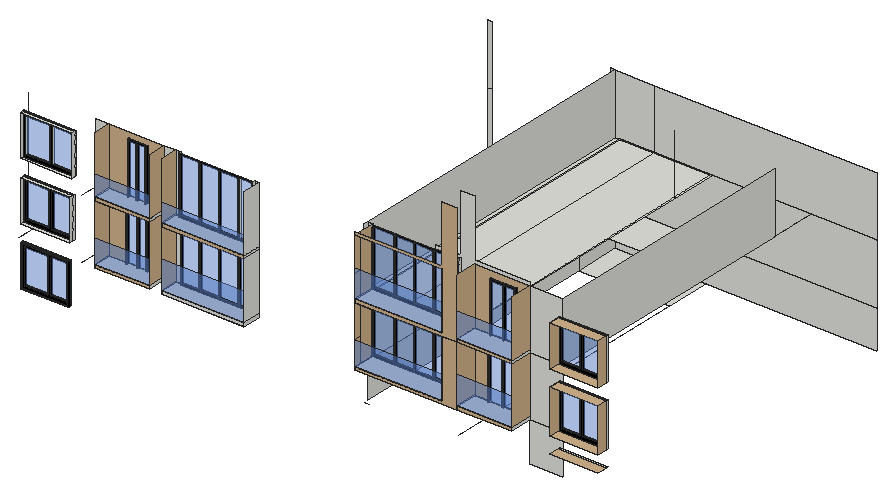
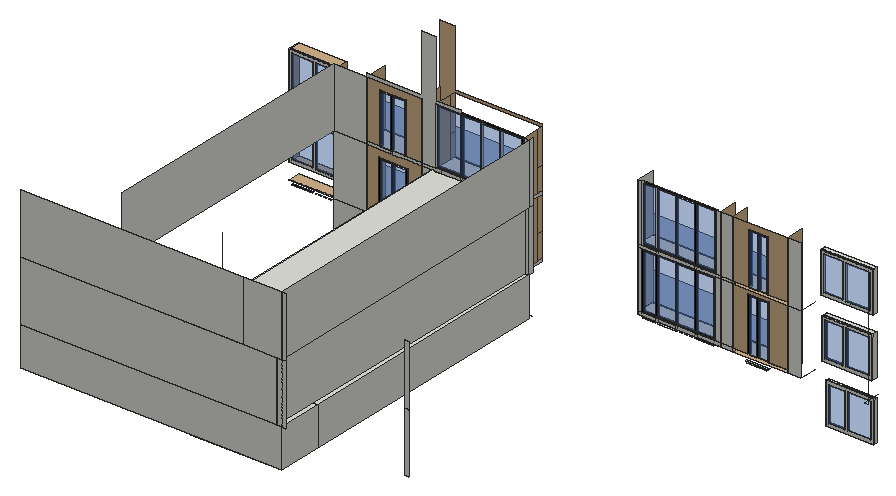
# SketchUp Ruby script. Lengths in inches.
U = 1.inch
M = Sketchup.active_model
def pt(a) = Geom::Point3d.new(a.map { |v| v * U })
def face(e, loops, mat)
  f = e.add_face(loops[0].map { |a| pt(a) })
  loops[1..].each { |l| e.add_face(l.map { |a| pt(a) }).erase! }
  f.material = f.back_material = mat if mat
  f
end
# faces: each face lists its corners as indices into pts; further lists are holes
def faces(e, pts, list, mat = nil) = list.each { |f| face(e, (f[0].is_a?(Array) ? f : [f]).map { |l| l.map { |i| pts[i] } }, mat) }
# xy, xz, yz: faces in a plane at the given z, y or x. An outline is a flat list of corners, or four numbers for a rectangle; further outlines are holes
def ring(l) = l.size == 4 ? [[l[0], l[1]], [l[2], l[1]], [l[2], l[3]], [l[0], l[3]]] : l.each_slice(2).to_a
def flat(e, list, mat, &to3) = list.each { |f| face(e, (f[0].is_a?(Array) ? f : [f]).map { |l| ring(l).map { |u, v| to3.(u, v) } }, mat) }
def xy(e, z, list, mat = nil) = flat(e, list, mat) { |x, y| [x, y, z] }
def xz(e, y, list, mat = nil) = flat(e, list, mat) { |x, z| [x, y, z] }
def yz(e, x, list, mat = nil) = flat(e, list, mat) { |y, z| [x, y, z] }
def lines(e, pts, list) = list.each { |a, b| e.add_line(pt(pts[a]), pt(pts[b])) }
# prism: a flat outline (further loops are holes) pulled along v
def prism(e, loops, v, mat = nil)
  f = face(e, loops, mat); d = Geom::Vector3d.new(v.map { |x| x * U })
  f.pushpull(f.normal.samedirection?(d) ? d.length : -d.length)
end
def box(e, o, s, mat = nil) = prism(e, [[o, [o[0] + s[0], o[1], o[2]], [o[0] + s[0], o[1] + s[1], o[2]], [o[0], o[1] + s[1], o[2]]]], [0, 0, s[2]], mat)
def at(x, y, z, deg = 0) = Geom::Transformation.translation(pt([x, y, z])) * Geom::Transformation.rotation(ORIGIN, Z_AXIS, deg.degrees)
def axes(o, x, y, z) = Geom::Transformation.new([*x, 0, *y, 0, *z, 0, *pt(o).to_a, 1])
def part(name) = M.definitions.add(name)
# library, detail: a bought-in or finely detailed component or shape, given as its bounding box
def library(name, o, s) = part(name).tap { |d| box(d.entities, o, s) }
def detail(e, o, s) = box(e.add_group.entities, o, s)
def put(e, d, t, mat = nil) = e.add_instance(d, t).tap { |i| i.material = mat if mat }
def group(e, t, mat = nil) = e.add_group.tap { |g| g.transformation = t; g.material = mat if mat }.entities
root = M.entities
M.materials.add("[0035_Tan]").color = [210, 180, 140]
M.materials.add("[0137_Black]").color = [0, 0, 0]
M.materials.add("[Translucent Glass Blue]").color = [100, 149, 237]
M.materials["[Translucent Glass Blue]"].alpha = 0.5
xy(root,157.15,[[83.625,162.2,178.82,165.57],[83.625,165.57,178.82,168.57]])
xy(root,163.15,[[89.625,165.57,135,168.57],[140.93,165.57,172.82,168.57]],"[0137_Black]")
xy(root,168.8125,[[737.47,731.95,917.4,821.88]])
xy(root,226.47,[[1141.77,183.2,1177.52,186.2],[1183.52,183.2,1225.27,186.2]],"[0137_Black]")
xy(root,229.5625,[[985.28,204.2,1008.35,207.2],[1011.35,204.2,1031.41,207.2]],"[0137_Black]")
xy(root,232.4,[[89.625,165.57,135,168.57],[140.93,165.57,172.82,168.57]])
xy(root,232.47,[[1135.77,183.2,1231.27,186.2]])
xy(root,232.47,[[1135.77,162.2,1231.27,183.2]],"[0035_Tan]")
xy(root,232.5625,[[982.28,204.2,1034.41,207.2]],"[0137_Black]")
xy(root,235.3125,[[271.43,195.2,290.12,198.2],[292.87,195.2,311.93,198.2]])
xy(root,238.3125,[[268.43,195.2,314.93,198.2]])
xy(root,238.4,[[83.625,162.2,178.82,165.57],[83.625,165.57,178.82,168.57]])
xy(root,243,[[415.22,195.2,451.16,198.2],[454.16,195.2,484.28,198.2],[484.28,195.2,489.53,198.2],[492.53,195.2,517.76,198.2]])
xy(root,243,[[378.57,195.2,412.22,198.2],[751.75,204.2,793,207.2],[796,204.2,831.1875,207.2],[834.1875,204.2,870.375,207.2],[873.375,204.2,911.73,207.2],
  [911.73,204.2,918.86,207.2]],"[0137_Black]")
xy(root,246,[[364.125,162.2,364.125,198.2,375.57,198.2,375.57,195.2,520.76,195.2,520.76,198.2,528.5625,198.2,528.5625,162.2],[921.86,162.2,930.34,199.63],[930.34,162.2,950.28,199.63],[375.57,195.2,412.22,198.2],[412.22,195.2,415.22,198.2],
  [415.22,195.2,451.16,198.2],[451.16,195.2,454.16,198.2],[454.16,195.2,489.53,198.2],[489.53,195.2,492.53,198.2],[492.53,195.2,520.76,198.2],
  [737.47,198.2,748.75,207.2],[921.86,199.63,930.34,207.2],[930.34,199.63,950.28,207.2],[748.75,204.2,793,207.2],[793,204.2,796,207.2],
  [796,204.2,831.1875,207.2],[831.1875,204.2,834.1875,207.2],[834.1875,204.2,870.375,207.2],[870.375,204.2,873.375,207.2],[873.375,204.2,911.73,207.2],
  [911.73,204.2,921.86,207.2],[737.47,207.2,746.47,731.95],[737.47,731.95,746.47,821.88],[746.47,731.95,930.34,821.88]])
xy(root,246,[[231.59,162.2,340.0625,198.2],[748.75,162.2,921.86,204.2],[950.28,162.2,1060.15,207.2]],"[0035_Tan]")
xy(root,252,[[231.59,162.2,340.0625,162.2,340.0625,198.2,309.85,198.2,309.85,195.2,306.85,195.2,306.85,198.2,292.57,198.2,292.57,195.2,288.7,195.2,288.7,198.2,270.54,198.2,270.54,195.2,267.54,195.2,267.54,198.2,231.59,198.2],[364.125,162.2,528.5625,162.2,528.5625,198.2,520.39,198.2,520.39,195.2,375.32,195.2,375.32,198.2,364.125,198.2],[748.75,162.2,921.86,204.2],[950.28,162.2,1060.15,162.2,1060.15,207.2,1035.75,207.2,1035.75,204.2,1032.75,204.2,1032.75,207.2,1010.53,207.2,1010.53,204.2,1007.53,204.2,1007.53,207.2,982.31,207.2,982.31,204.2,979.31,204.2,979.31,207.2,950.28,207.2],[375.32,195.2,412.22,198.2],
  [412.22,195.2,415.22,198.2],[415.22,195.2,451.16,198.2],[451.16,195.2,454.16,198.2],[454.16,195.2,489.53,198.2],[489.53,195.2,492.53,198.2],
  [492.53,195.2,520.39,198.2],[748.75,204.2,793,207.2],[793,204.2,796,207.2],[796,204.2,831.1875,207.2],[831.1875,204.2,834.1875,207.2],
  [834.1875,204.2,870.375,207.2],[870.375,204.2,873.375,207.2],[873.375,204.2,911.73,207.2],[911.73,204.2,921.86,207.2],[979.31,204.2,982.31,207.2],
  [1007.53,204.2,1008.35,207.2],[1008.35,204.2,1010.53,207.2],[1032.75,204.2,1035.75,207.2]])
xy(root,255,[[378.32,195.2,412.22,198.2],[415.22,195.2,451.16,198.2],[454.16,195.2,489.53,198.2],[492.53,195.2,517.39,198.2],[751.75,204.2,793,207.2],
  [796,204.2,831.1875,207.2],[834.1875,204.2,870.375,207.2],[873.375,204.2,911.73,207.2],[911.73,204.2,918.86,207.2]],"[0137_Black]")
xy(root,264.66,[[1135.77,183.2,1231.27,186.2]])
xy(root,264.66,[[1135.77,162.2,1231.27,183.2]],"[0035_Tan]")
xy(root,270.66,[[1141.77,183.2,1177.52,186.2],[1183.52,183.2,1225.27,186.2]],"[0137_Black]")
xy(root,273.03,[[83.625,162.2,182.53,169.82],[83.625,169.82,182.53,172.82]])
xy(root,279.03,[[89.625,169.82,134.93,172.82],[140.93,169.82,176.53,172.82]],"[0137_Black]")
xy(root,345.78,[[1141.77,183.2,1177.52,186.2],[1183.52,183.2,1225.27,186.2]],"[0137_Black]")
xy(root,348.1875,[[982.31,204.2,1007.53,207.2],[1010.53,204.2,1032.75,207.2]])
xy(root,348.28,[[89.625,169.82,134.93,172.82],[140.93,169.82,176.53,172.82]])
xy(root,351.1875,[[979.31,204.2,1035.75,207.2]],"[0137_Black]")
xy(root,351.78,[[1135.77,183.2,1231.27,186.2]])
xy(root,351.78,[[1135.77,162.2,1231.27,183.2]],"[0035_Tan]")
xy(root,354.28,[[83.625,162.2,182.53,169.82],[83.625,169.82,182.53,172.82]])
xy(root,356.5625,[[270.54,195.2,288.7,198.2],[292.57,195.2,306.85,198.2]],"[0137_Black]")
xy(root,359.5625,[[267.54,195.2,309.85,198.2]],"[0137_Black]")
xy(root,363,[[378.32,195.2,412.22,198.2],[415.22,195.2,451.16,198.2],[454.16,195.2,484.28,198.2],[484.28,195.2,489.53,198.2],[492.53,195.2,517.39,198.2],
  [751.75,204.2,793,207.2],[796,204.2,814.9,207.2],[814.9,204.2,831.1875,207.2],[834.1875,204.2,870.375,207.2],[873.375,204.2,911.73,207.2],
  [911.73,204.2,918.86,207.2]],"[0137_Black]")
xy(root,366,[[921.86,162.2,928.15,207.2],[928.15,162.2,930.34,207.2],[930.34,162.2,950.28,207.2],[375.32,195.2,412.22,198.2],[412.22,195.2,415.22,198.2],
  [415.22,195.2,489.53,198.2],[489.53,195.2,492.53,198.2],[492.53,195.2,520.39,198.2],[748.75,204.2,793,207.2],[793,204.2,796,207.2],
  [796,204.2,814.9,207.2],[814.9,204.2,831.1875,207.2],[831.1875,204.2,834.1875,207.2],[834.1875,204.2,870.375,207.2],[870.375,204.2,873.375,207.2],
  [873.375,204.2,911.73,207.2],[911.73,204.2,921.86,207.2],[737.47,207.2,746.47,821.88],[746.47,207.2,814.9,821.88],[814.9,207.2,928.15,821.88],
  [928.15,207.2,930.34,731.95],[928.15,731.95,930.34,821.88]])
xy(root,366,[[231.59,162.2,340.0625,198.2],[364.125,162.2,364.125,198.2,375.32,198.2,375.32,195.2,520.39,195.2,520.39,198.2,528.5625,198.2,528.5625,162.2],[748.75,162.2,921.86,174.2],[950.28,162.2,1060.15,207.2],[748.75,174.2,921.86,204.2]],"[0035_Tan]")
xy(root,372,[[231.59,162.2,340.0625,162.2,340.0625,198.2,308.39,198.2,308.39,195.2,305.39,195.2,305.39,198.2,290.52,198.2,290.52,195.2,287.52,195.2,287.52,198.2,272.83,198.2,272.83,195.2,269.83,195.2,269.83,198.2,231.59,198.2],[364.125,162.2,528.5625,162.2,528.5625,198.2,519.88,198.2,519.88,195.2,372.82,195.2,372.82,198.2,364.125,198.2],[748.75,162.2,921.86,204.2],[950.28,162.2,1060.15,162.2,1060.15,207.2,1034.41,207.2,1034.41,204.2,1031.41,204.2,1031.41,207.2,1011.35,207.2,1011.35,204.2,1008.35,204.2,1008.35,207.2,985.28,207.2,985.28,204.2,982.28,204.2,982.28,207.2,950.28,207.2],[372.82,195.2,412.22,198.2],
  [412.22,195.2,415.22,198.2],[415.22,195.2,489.53,198.2],[489.53,195.2,492.53,198.2],[492.53,195.2,519.88,198.2],[748.75,204.2,793,207.2],
  [793,204.2,796,207.2],[796,204.2,831.1875,207.2],[831.1875,204.2,834.1875,207.2],[834.1875,204.2,870.375,207.2],[870.375,204.2,873.375,207.2],
  [873.375,204.2,911.73,207.2],[911.73,204.2,921.86,207.2],[982.28,204.2,985.28,207.2],[1008.35,204.2,1011.35,207.2],[1031.41,204.2,1034.41,207.2]])
xy(root,375,[[911.73,204.2,918.86,207.2]])
xy(root,375,[[375.82,195.2,412.22,198.2],[415.22,195.2,451.16,198.2],[454.16,195.2,489.53,198.2],[492.53,195.2,516.88,198.2],[751.75,204.2,793,207.2],
  [796,204.2,831.1875,207.2],[834.1875,204.2,870.375,207.2],[873.375,204.2,911.73,207.2]],"[0137_Black]")
xy(root,383.34,[[1135.77,183.2,1231.27,186.2]])
xy(root,383.34,[[1135.77,162.2,1231.27,183.2]],"[0035_Tan]")
xy(root,388.91,[[83.625,162.2,186.23,168.95],[83.625,168.95,186.23,171.95]])
xy(root,389.34,[[1141.77,183.2,1177.52,186.2],[1183.52,183.2,1225.27,186.2]],"[0137_Black]")
xy(root,394.91,[[89.625,168.95,137.0625,171.95],[142.78,168.95,180.23,171.95]])
xy(root,460.47,[[1141.77,183.2,1177.52,186.2],[1183.52,183.2,1225.27,186.2]],"[0137_Black]")
xy(root,464.16,[[89.625,168.95,137.0625,171.95],[142.78,168.95,180.23,171.95]])
xy(root,466.47,[[1135.77,183.2,1231.27,186.2]])
xy(root,466.47,[[1135.77,162.2,1231.27,183.2]],"[0035_Tan]")
xy(root,468.9375,[[985.28,204.2,1008.35,207.2],[1011.35,204.2,1031.41,207.2]])
xy(root,470.16,[[83.625,162.2,186.23,168.95],[83.625,168.95,186.23,171.95]])
xy(root,471.9375,[[982.28,204.2,1034.41,207.2]])
xy(root,471.9375,[[272.83,195.2,287.52,198.2],[290.52,195.2,305.39,198.2]],"[0137_Black]")
xy(root,474.9375,[[269.83,195.2,308.39,198.2]],"[0137_Black]")
xy(root,483,[[375.82,195.2,412.22,198.2],[415.22,195.2,451.16,198.2],[454.16,195.2,484.28,198.2],[484.28,195.2,489.53,198.2],[492.53,195.2,516.88,198.2]])
xy(root,483,[[751.75,204.2,793,207.2],[796,204.2,814.9,207.2],[814.9,204.2,831.1875,207.2],[834.1875,204.2,870.375,207.2],[873.375,204.2,911.73,207.2],
  [911.73,204.2,918.86,207.2]],"[0137_Black]")
xz(root,162.2,[[364.125,246,528.5625,252]])
xz(root,162.2,[[231.59,246,340.0625,252],[748.75,246,950.28,246,950.28,366,921.86,366,921.86,252,748.75,252],[950.28,246,1060.15,252],[231.59,366,340.0625,372],[364.125,366,528.5625,372],
  [748.75,366,950.28,366,950.28,606,921.86,606,921.86,492,748.75,492,748.75,486,921.86,486,921.86,372,748.75,372],[950.28,366,1060.15,372]],"[0035_Tan]")
xz(root,162.2,[[231.59,252,340.0625,299.77],[364.125,252,528.5625,309],[748.75,252,921.86,300.08],[950.28,252,1060.15,309],[231.59,372,340.0625,413.33],
  [364.125,372,528.5625,409.78],[748.75,372,921.86,428],[950.28,372,1060.15,422.45]],"[Translucent Glass Blue]")
xz(root,165.57,[[[83.625,157.15,178.82,238.4],[89.625,163.15,135,232.4],[140.93,163.15,172.82,232.4]]],"[0137_Black]")
xz(root,168.57,[[[83.625,157.15,178.82,238.4],[89.625,163.15,135,232.4],[140.93,163.15,172.82,232.4]]])
xz(root,168.57,[[89.625,163.15,135,232.4],[140.93,163.15,172.82,232.4]],"[Translucent Glass Blue]")
xz(root,168.95,[[[83.625,388.91,186.23,470.16],[89.625,394.91,137.0625,464.16],[142.78,394.91,180.23,464.16]]],"[0137_Black]")
xz(root,169.82,[[[83.625,273.03,182.53,354.28],[89.625,279.03,134.93,348.28],[140.93,279.03,176.53,348.28]]],"[0137_Black]")
xz(root,171.95,[[[83.625,388.91,186.23,470.16],[89.625,394.91,137.0625,464.16],[142.78,394.91,180.23,464.16]]])
xz(root,171.95,[[89.625,394.91,137.0625,464.16],[142.78,394.91,180.23,464.16]],"[Translucent Glass Blue]")
xz(root,172.82,[[[83.625,273.03,182.53,354.28],[89.625,279.03,134.93,348.28],[140.93,279.03,176.53,348.28]]])
xz(root,172.82,[[89.625,279.03,134.93,348.28],[140.93,279.03,176.53,348.28]],"[Translucent Glass Blue]")
xz(root,183.2,[[[1135.77,264.66,1231.27,351.78],[1183.52,270.66,1225.27,345.78],[1141.77,270.66,1177.52,345.78]],[[1135.77,383.34,1231.27,466.47],[1183.52,389.34,1225.27,460.47],[1141.77,389.34,1177.52,460.47]]],"[0137_Black]")
xz(root,186.2,[[[1135.77,264.66,1231.27,351.78],[1183.52,270.66,1225.27,345.78],[1141.77,270.66,1177.52,345.78]],[[1135.77,383.34,1231.27,466.47],[1183.52,389.34,1225.27,460.47],[1141.77,389.34,1177.52,460.47]]])
xz(root,186.2,[[1141.77,270.66,1177.52,345.78],[1183.52,270.66,1225.27,345.78],[1141.77,389.34,1177.52,460.47],[1183.52,389.34,1225.27,460.47]],"[Translucent Glass Blue]")
xz(root,195.2,[[267.54,252,270.54,252,270.54,356.5625,288.7,356.5625,288.7,252,292.57,252,292.57,356.5625,306.85,356.5625,306.85,252,309.85,252,309.85,359.5625,267.54,359.5625],[[375.32,252,520.39,366],[415.22,255,451.16,363],[454.16,255,489.53,363],[378.32,255,412.22,363],[492.53,255,517.39,363]],[269.83,372,272.83,372,272.83,471.9375,287.52,471.9375,287.52,372,290.52,372,290.52,471.9375,305.39,471.9375,305.39,372,308.39,372,308.39,474.9375,269.83,474.9375],[[372.82,372,519.88,486],[375.82,375,412.22,483],[415.22,375,451.16,483],[454.16,375,489.53,483],[492.53,375,516.88,483]]],"[0137_Black]")
xz(root,198.2,[[204.84,246,231.59,366],[340.0625,246,364.125,252],[364.125,246,412.22,252],[412.22,246,415.22,252],[415.22,246,451.16,252],
  [451.16,246,454.16,252],[454.16,246,489.53,252],[489.53,246,492.53,252],[492.53,246,528.5625,252],[340.0625,252,364.125,366],
  [364.125,252,375.32,366],[520.39,252,528.5625,366],[204.84,366,231.59,486],[340.0625,366,364.125,372],[364.125,366,412.22,372],
  [412.22,366,415.22,372],[415.22,366,489.53,372],[489.53,366,492.53,372],[492.53,366,528.5625,372],[340.0625,372,364.125,486],
  [364.125,372,372.82,486],[519.88,372,528.5625,486]])
xz(root,198.2,[[231.59,252,267.54,252,267.54,359.5625,309.85,359.5625,309.85,252,340.0625,252,340.0625,366,231.59,366],[231.59,372,269.83,372,269.83,474.9375,308.39,474.9375,308.39,372,340.0625,372,340.0625,486,231.59,486]],"[0035_Tan]")
xz(root,198.2,[[270.54,252,288.7,356.5625],[292.57,252,306.85,356.5625],[378.32,255,412.22,363],[415.22,255,451.16,363],[454.16,255,489.53,363],
  [492.53,255,517.39,363],[272.83,372,287.52,471.9375],[290.52,372,305.39,471.9375],[375.82,375,412.22,483],[415.22,375,451.16,483],
  [454.16,375,489.53,483],[492.53,375,516.88,483]],"[Translucent Glass Blue]")
xz(root,204.2,[[[748.75,252,921.86,366],[873.375,255,918.86,363],[751.75,255,793,363],[834.1875,255,870.375,363],[796,255,831.1875,363]],[979.31,252,982.31,252,982.31,348.1875,1007.53,348.1875,1007.53,252,1010.53,252,1010.53,348.1875,1032.75,348.1875,1032.75,252,1035.75,252,1035.75,351.1875,979.31,351.1875],[[748.75,372,921.86,486],[873.375,375,918.86,483],[751.75,375,793,483],[834.1875,375,870.375,483],[796,375,831.1875,483]],[982.28,372,985.28,372,985.28,468.9375,1008.35,468.9375,1008.35,372,1011.35,372,1011.35,468.9375,1031.41,468.9375,1031.41,372,1034.41,372,1034.41,471.9375,982.28,471.9375]],"[0137_Black]")
xz(root,207.2,[[1060.15,168.8125,1125.97,246],[737.47,246,746.47,366],[746.47,246,748.75,366],[748.75,246,793,252],[793,246,796,252],
  [796,246,831.1875,252],[831.1875,246,834.1875,252],[834.1875,246,870.375,252],[870.375,246,873.375,252],[873.375,246,911.73,252],
  [911.73,246,911.73,252,921.86,252,921.86,366,950.28,366,950.28,246],[950.28,246,1008.35,252],[1008.35,246,1011.35,252],[1011.35,246,1060.15,252],[1060.15,246,1125.97,366],
  [737.47,366,748.75,486],[748.75,366,793,372],[793,366,796,372],[796,366,831.1875,372],[831.1875,366,834.1875,372],
  [834.1875,366,870.375,372],[870.375,366,873.375,372],[873.375,366,911.73,372],[911.73,366,950.28,372],[950.28,366,1008.35,372],
  [1008.35,366,1011.35,372],[1011.35,366,1060.15,372],[1060.15,366,1125.97,486],[921.86,372,950.28,372,950.28,486,1060.15,486,1060.15,492,950.28,492,950.28,606,921.86,606,921.86,492,873.375,492,873.375,486,921.86,486]])
xz(root,207.2,[[950.28,252,979.31,252,979.31,351.1875,1035.75,351.1875,1035.75,252,1060.15,252,1060.15,366,950.28,366],[950.28,372,982.28,372,982.28,471.9375,1034.41,471.9375,1034.41,372,1060.15,372,1060.15,486,950.28,486]],"[0035_Tan]")
xz(root,207.2,[[982.31,252,1007.53,348.1875],[1010.53,252,1032.75,348.1875],[751.75,255,793,363],[796,255,831.1875,363],[834.1875,255,870.375,363],
  [873.375,255,918.86,363],[985.28,372,1008.35,468.9375],[1011.35,372,1031.41,468.9375],[751.75,375,793,483],[796,375,831.1875,483],
  [834.1875,375,870.375,483],[873.375,375,918.86,483]],"[Translucent Glass Blue]")
xz(root,821.88,[[737.47,168.8125,1256.59,246],[484.28,246,493.28,366],[728.47,246,737.47,366],[737.47,246,746.47,366],[746.47,246,1256.59,366],
  [484.28,366,493.28,486],[728.47,366,737.47,486],[737.47,366,814.9,486],[814.9,366,1256.59,486]])
yz(root,83.625,[[162.2,157.15,165.57,238.4],[165.57,157.15,168.57,238.4],[162.2,273.03,169.82,354.28],[169.82,273.03,172.82,354.28],[162.2,388.91,168.95,470.16],
  [168.95,388.91,171.95,470.16]])
yz(root,89.625,[[168.95,394.91,171.95,464.16]])
yz(root,89.625,[[165.57,163.15,168.57,232.4],[169.82,279.03,172.82,348.28]],"[0137_Black]")
yz(root,134.93,[[169.82,279.03,172.82,348.28]],"[0137_Black]")
yz(root,135,[[165.57,163.15,168.57,232.4]],"[0137_Black]")
yz(root,137.0625,[[168.95,394.91,171.95,464.16]])
yz(root,140.93,[[165.57,163.15,168.57,232.4],[169.82,279.03,172.82,348.28]],"[0137_Black]")
yz(root,142.78,[[168.95,394.91,171.95,464.16]])
yz(root,172.82,[[165.57,163.15,168.57,232.4]],"[0137_Black]")
yz(root,176.53,[[169.82,279.03,172.82,348.28]],"[0137_Black]")
yz(root,178.82,[[165.57,157.15,168.57,238.4]])
yz(root,178.82,[[162.2,157.15,165.57,238.4]],"[0137_Black]")
yz(root,180.23,[[168.95,394.91,171.95,464.16]])
yz(root,182.53,[[162.2,273.03,169.82,354.28],[169.82,273.03,172.82,354.28]])
yz(root,186.23,[[162.2,388.91,168.95,470.16],[168.95,388.91,171.95,470.16]])
yz(root,231.59,[[162.2,246,198.2,252],[162.2,366,198.2,372]])
yz(root,231.59,[[162.2,252,198.2,366],[162.2,372,198.2,486]],"[0035_Tan]")
yz(root,267.54,[[195.2,252,198.2,359.5625]],"[0137_Black]")
yz(root,269.83,[[195.2,372,198.2,474.9375]],"[0137_Black]")
yz(root,270.54,[[195.2,252,198.2,356.5625]],"[0137_Black]")
yz(root,272.83,[[195.2,372,198.2,375]])
yz(root,272.83,[[195.2,375,198.2,471.9375]],"[0137_Black]")
yz(root,287.52,[[195.2,372,198.2,471.9375]],"[0137_Black]")
yz(root,288.7,[[195.2,252,198.2,356.5625]],"[0137_Black]")
yz(root,290.52,[[195.2,372,198.2,471.9375]],"[0137_Black]")
yz(root,292.57,[[195.2,252,198.2,356.5625]],"[0137_Black]")
yz(root,305.39,[[195.2,372,198.2,375]])
yz(root,305.39,[[195.2,375,198.2,471.9375]],"[0137_Black]")
yz(root,306.85,[[195.2,252,198.2,356.5625]],"[0137_Black]")
yz(root,308.39,[[195.2,372,198.2,474.9375]],"[0137_Black]")
yz(root,309.85,[[195.2,252,198.2,359.5625]],"[0137_Black]")
yz(root,340.0625,[[162.2,246,198.2,252],[162.2,366,198.2,372]])
yz(root,340.0625,[[162.2,252,198.2,366],[162.2,372,198.2,486]],"[0035_Tan]")
yz(root,364.125,[[162.2,246,198.2,252],[162.2,366,198.2,372]])
yz(root,364.125,[[162.2,252,198.2,366],[162.2,372,198.2,486]],"[0035_Tan]")
yz(root,372.82,[[195.2,372,198.2,486]])
yz(root,375.32,[[195.2,252,198.2,366]],"[0137_Black]")
yz(root,375.82,[[195.2,375,198.2,483]],"[0137_Black]")
yz(root,378.32,[[195.2,255,198.2,363]],"[0137_Black]")
yz(root,412.22,[[195.2,255,198.2,363],[195.2,375,198.2,483]],"[0137_Black]")
yz(root,415.22,[[195.2,255,198.2,363],[195.2,375,198.2,483]],"[0137_Black]")
yz(root,451.16,[[195.2,255,198.2,363],[195.2,375,198.2,483]],"[0137_Black]")
yz(root,454.16,[[195.2,255,198.2,363],[195.2,375,198.2,483]],"[0137_Black]")
yz(root,489.53,[[195.2,255,198.2,363],[195.2,375,198.2,483]],"[0137_Black]")
yz(root,492.53,[[195.2,375,198.2,483]])
yz(root,492.53,[[195.2,255,198.2,363]],"[0137_Black]")
yz(root,516.88,[[195.2,375,198.2,483]],"[0137_Black]")
yz(root,517.39,[[195.2,255,198.2,363]],"[0137_Black]")
yz(root,519.88,[[195.2,372,198.2,486]])
yz(root,520.39,[[195.2,252,198.2,366]],"[0137_Black]")
yz(root,528.5625,[[162.2,246,198.2,252],[162.2,252,198.2,366],[162.2,366,198.2,372],[162.2,372,198.2,486]])
yz(root,737.47,[[207.2,168.8125,731.95,246],[731.95,168.8125,821.88,246],[198.2,246,207.2,366],[198.2,366,207.2,486],[207.2,366,821.88,486]])
yz(root,746.47,[[207.2,246,821.88,366]])
yz(root,748.75,[[162.2,246,198.2,252],[198.2,246,207.2,252],[204.2,252,207.2,366],[162.2,366,198.2,372],[198.2,366,207.2,372],
  [204.2,372,207.2,486]])
yz(root,748.75,[[162.2,252,174.2,300.08],[174.2,252,204.2,366],[162.2,300.08,174.2,366],[162.2,372,174.2,416.46],[174.2,372,204.2,486],
  [162.2,416.46,174.2,486]],"[0035_Tan]")
yz(root,751.75,[[204.2,255,207.2,363],[204.2,375,207.2,483]],"[0137_Black]")
yz(root,793,[[204.2,375,207.2,483]])
yz(root,793,[[204.2,255,207.2,363]],"[0137_Black]")
yz(root,796,[[204.2,255,207.2,363],[204.2,375,207.2,483]],"[0137_Black]")
yz(root,831.1875,[[204.2,375,207.2,483]])
yz(root,831.1875,[[204.2,255,207.2,363]],"[0137_Black]")
yz(root,834.1875,[[204.2,255,207.2,363],[204.2,375,207.2,483]],"[0137_Black]")
yz(root,870.375,[[204.2,255,207.2,363],[204.2,375,207.2,483]],"[0137_Black]")
yz(root,873.375,[[204.2,255,207.2,363],[204.2,375,207.2,483]],"[0137_Black]")
yz(root,918.86,[[204.2,255,207.2,363],[204.2,375,207.2,483]],"[0137_Black]")
yz(root,921.86,[[204.2,252,207.2,366],[204.2,372,207.2,486]])
yz(root,921.86,[[162.2,252,174.2,300.08],[174.2,252,204.2,366],[162.2,300.08,174.2,366],[162.2,372,174.2,416.46],[174.2,372,204.2,486],
  [162.2,416.46,174.2,486]],"[0035_Tan]")
yz(root,950.28,[[162.2,246,207.2,252],[162.2,366,207.2,372]])
yz(root,950.28,[[162.2,252,207.2,366],[162.2,372,207.2,486]],"[0035_Tan]")
yz(root,979.31,[[204.2,252,207.2,351.1875]],"[0137_Black]")
yz(root,982.28,[[204.2,372,207.2,372.3125]])
yz(root,982.28,[[204.2,372.3125,207.2,471.9375]],"[0137_Black]")
yz(root,982.31,[[204.2,252,207.2,255]])
yz(root,982.31,[[204.2,255,207.2,348.1875]],"[0137_Black]")
yz(root,985.28,[[204.2,372,207.2,375.3125],[204.2,375.3125,207.2,468.9375]],"[0137_Black]")
yz(root,1007.53,[[204.2,252,207.2,348.1875]],"[0137_Black]")
yz(root,1008.35,[[204.2,372,207.2,468.9375]],"[0137_Black]")
yz(root,1010.53,[[204.2,252,207.2,348.1875]],"[0137_Black]")
yz(root,1011.35,[[204.2,372,207.2,468.9375]],"[0137_Black]")
yz(root,1031.41,[[204.2,372,207.2,375.3125],[204.2,375.3125,207.2,468.9375]],"[0137_Black]")
yz(root,1032.75,[[204.2,252,207.2,255]])
yz(root,1032.75,[[204.2,255,207.2,348.1875]],"[0137_Black]")
yz(root,1034.41,[[204.2,372,207.2,372.3125]])
yz(root,1034.41,[[204.2,372.3125,207.2,471.9375]],"[0137_Black]")
yz(root,1035.75,[[204.2,252,207.2,351.1875]],"[0137_Black]")
yz(root,1060.15,[[162.2,246,207.2,252],[162.2,366,207.2,372]])
yz(root,1060.15,[[162.2,252,207.2,366],[162.2,372,207.2,486]],"[0035_Tan]")
yz(root,1125.97,[[207.2,366,731.95,486]])
yz(root,1135.77,[[183.2,264.66,186.2,351.78],[183.2,383.34,186.2,466.47]])
yz(root,1135.77,[[162.2,264.66,183.2,351.78],[162.2,383.34,183.2,466.47]],"[0035_Tan]")
yz(root,1141.77,[[183.2,270.66,186.2,345.78],[183.2,389.34,186.2,460.47]],"[0137_Black]")
yz(root,1177.52,[[183.2,270.66,186.2,345.78],[183.2,389.34,186.2,460.47]],"[0137_Black]")
yz(root,1183.52,[[183.2,270.66,186.2,345.78],[183.2,389.34,186.2,460.47]],"[0137_Black]")
yz(root,1225.27,[[183.2,270.66,186.2,345.78],[183.2,389.34,186.2,460.47]],"[0137_Black]")
yz(root,1231.27,[[183.2,264.66,186.2,351.78],[183.2,383.34,186.2,466.47]])
yz(root,1231.27,[[162.2,264.66,183.2,351.78],[162.2,383.34,183.2,466.47]],"[0035_Tan]")
p = [[1125.97,731.95,366],[1125.97,821.88,366],[69.9,198.2,486],[69.9,198.2,246],[928.15,731.95,486],[928.15,731.95,366],
  [917.4,731.95,168.8125],[917.4,207.2,168.8125],[737.47,198.2,168.8125],[748.75,198.2,168.8125],[204.84,198.2,366],[204.84,162.2,366],
  [79.47,198.2,246],[204.84,198.2,246],[204.84,162.2,246],[79.47,162.2,246]]
lines(root,p,[[0,1],[2,3],[4,5],[6,7],[8,9],[10,11],[3,12],[13,14],[12,15]])
